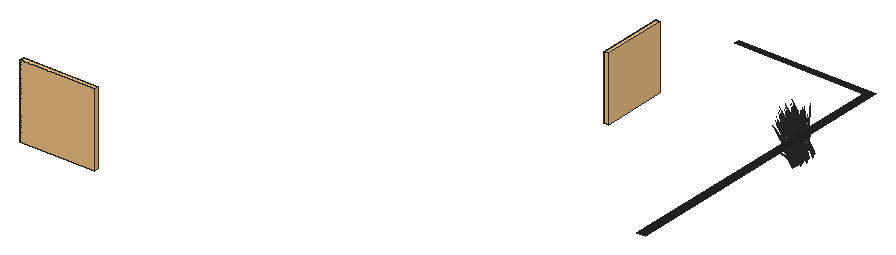
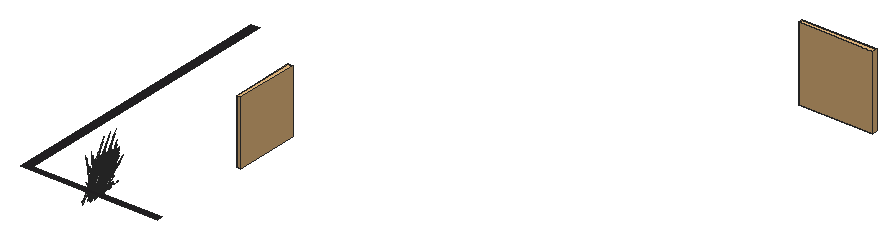
# SketchUp Ruby script. Lengths in inches.
U = 1.inch
M = Sketchup.active_model
def pt(a) = Geom::Point3d.new(a.map { |v| v * U })
def face(e, loops, mat)
  f = e.add_face(loops[0].map { |a| pt(a) })
  loops[1..].each { |l| e.add_face(l.map { |a| pt(a) }).erase! }
  f.material = f.back_material = mat if mat
  f
end
# faces: each face lists its corners as indices into pts; further lists are holes
def faces(e, pts, list, mat = nil) = list.each { |f| face(e, (f[0].is_a?(Array) ? f : [f]).map { |l| l.map { |i| pts[i] } }, mat) }
# xy, xz, yz: faces in a plane at the given z, y or x. An outline is a flat list of corners, or four numbers for a rectangle; further outlines are holes
def ring(l) = l.size == 4 ? [[l[0], l[1]], [l[2], l[1]], [l[2], l[3]], [l[0], l[3]]] : l.each_slice(2).to_a
def flat(e, list, mat, &to3) = list.each { |f| face(e, (f[0].is_a?(Array) ? f : [f]).map { |l| ring(l).map { |u, v| to3.(u, v) } }, mat) }
def xy(e, z, list, mat = nil) = flat(e, list, mat) { |x, y| [x, y, z] }
def xz(e, y, list, mat = nil) = flat(e, list, mat) { |x, z| [x, y, z] }
def yz(e, x, list, mat = nil) = flat(e, list, mat) { |y, z| [x, y, z] }
def lines(e, pts, list) = list.each { |a, b| e.add_line(pt(pts[a]), pt(pts[b])) }
# prism: a flat outline (further loops are holes) pulled along v
def prism(e, loops, v, mat = nil)
  f = face(e, loops, mat); d = Geom::Vector3d.new(v.map { |x| x * U })
  f.pushpull(f.normal.samedirection?(d) ? d.length : -d.length)
end
def box(e, o, s, mat = nil) = prism(e, [[o, [o[0] + s[0], o[1], o[2]], [o[0] + s[0], o[1] + s[1], o[2]], [o[0], o[1] + s[1], o[2]]]], [0, 0, s[2]], mat)
def at(x, y, z, deg = 0) = Geom::Transformation.translation(pt([x, y, z])) * Geom::Transformation.rotation(ORIGIN, Z_AXIS, deg.degrees)
def axes(o, x, y, z) = Geom::Transformation.new([*x, 0, *y, 0, *z, 0, *pt(o).to_a, 1])
def part(name) = M.definitions.add(name)
# library, detail: a bought-in or finely detailed component or shape, given as its bounding box
def library(name, o, s) = part(name).tap { |d| box(d.entities, o, s) }
def detail(e, o, s) = box(e.add_group.entities, o, s)
def put(e, d, t, mat = nil) = e.add_instance(d, t).tap { |i| i.material = mat if mat }
def group(e, t, mat = nil) = e.add_group.tap { |g| g.transformation = t; g.material = mat if mat }.entities
root = M.entities
M.materials.add("LightPink_Translucent").color = [144, 107, 117]
M.materials["LightPink_Translucent"].alpha = 0.75
M.materials.add("Marble_07_1K").color = [36, 34, 36]
c1 = library("mesh-163",[-551.08,-704.17,-20.03],[1929.24,1401.85,86.96])
c2 = part("Group11")
put(c2.entities,c1,at(0,0,0))
c3 = part("blade")
p = [[2.15,0.21,22],[0,0.17,0],[0.09,0.45,0],[2.18,0.31,22],[2.29,0.31,22],[0.38,0.45,0],
  [2.48,0.24,33],[2.49,0.24,33],[2.48,0.22,33]]
faces(c3.entities,p,[[0,1,2,3],[4,5,2,3],[6,3,4,7],[8,0,3,6]])
c4 = part("seeds")
p = [[0.3,-0.1,1.38],[-0.01,-0.03,1.59],[-0.01,-0.03,0.03],[0.14,-0.07,-0.07],[0.29,-0.03,3],[0.15,0.01,3.11]]
faces(c4.entities,p,[[0,1,2,3],[1,0,4,5]],"LightPink_Translucent")
c5 = part("blade with seeds")
put(c5.entities,c3,at(0,0,0))
put(c5.entities,c4,axes([2.4,0.25,30.99],[1.5799,-0.05474,1.17369],[-0.12525,1.92788,0.29478],[-0.07173,-0.02425,1.56792]))
xy(root,300,[[699.71,144,706,144,706,360,603,360,603,356,699.71,356]],"Marble_07_1K")
put(root,c2,axes([385.5,9.94,323.29],[-0.02883,0,0],[0,0,0.03929],[0,0.03937,0]))
put(root,c2,axes([603.79,247.71,324.08],[0,0.02488,0],[0,0,0.0342],[0.03937,0,0]))
put(root,c5,axes([686.23,308.34,267.22],[0.14872,0.18332,1.42242],[-0.6872,0.15433,0.11501],[-0.15531,-0.28779,0.60807]))
put(root,c5,axes([686.68,306.86,267.91],[-0.01214,0.06844,1.47228],[-0.59861,0.24837,-0.13912],[-0.17615,-0.12696,0.26054]))
put(root,c5,axes([686.55,308.08,268.23],[0.72473,-0.14676,0.44623],[0.12578,0.57568,0.36794],[-0.17045,-0.16967,0.92337]))
put(root,c5,axes([685.84,307.56,266.3],[0.33937,0.19872,0.95334],[-0.49424,0.11946,0.70045],[-0.10575,-0.15273,0.20998]))
put(root,c5,axes([686.66,308.61,268.13],[-0.55475,-0.27598,-0.58968],[0.39425,-0.48361,0.07116],[-0.20099,-0.16478,0.83415]))
put(root,c5,axes([686.47,308.24,267.76],[-0.10048,-0.4599,-0.29394],[0.5744,-0.12144,0.37948],[-0.15428,-0.13179,0.72609]))
put(root,c5,axes([686.72,308.2,267.93],[0.29569,-0.36271,0.05337],[0.42107,0.21117,0.42015],[-0.13613,-0.11629,0.64067]))
put(root,c5,axes([685.23,308.91,267.22],[0.24166,0.09837,1.42242],[-0.50011,0.41269,0.11501],[-0.3117,-0.18617,0.60807]))
put(root,c5,axes([686.4,308.62,267.89],[-0.64198,0.13573,-0.42412],[-0.1123,-0.514,-0.32852],[-0.17243,-0.1473,0.81151]))
put(root,c5,axes([686.85,308.16,268.51],[-0.4342,0.54737,-0.11304],[-0.6288,-0.31535,-0.62743],[-0.21858,-0.15465,0.95337]))
put(root,c5,axes([685.1875,308.01,267.91],[-0.13998,-0.00403,1.45204],[-0.44565,0.40302,-0.22964],[-0.23779,-0.08235,0.11645]))
put(root,c5,axes([687.99,311.73,266.76],[0.56221,0.23024,1.25546],[-0.55078,0.49601,0.49647],[-0.2467,-0.29398,1.05249]))
put(root,c5,axes([686.81,308.62,268.19],[0.10048,0.4599,0.29394],[-0.5744,0.12144,-0.37948],[-0.15428,-0.13179,0.72609]))
put(root,c5,axes([685.09,308.92,268.23],[0.53728,-0.42137,0.44623],[0.46337,0.44748,0.36794],[-0.25207,-0.07773,0.92337]))
put(root,c5,axes([685.33,308.92,267.93],[0.03276,-0.43418,0.05337],[0.49468,0.0119,0.42015],[-0.18949,-0.04543,0.64067]))
put(root,c5,axes([685.14,309.05,267.76],[-0.37017,-0.35748,-0.29394],[0.42268,-0.3384,0.37948],[-0.21476,-0.05149,0.72609]))
put(root,c5,axes([685.53,309.29,268.13],[-0.65035,-0.01375,-0.58968],[0.04368,-0.5789,0.07116],[-0.27552,-0.06109,0.83415]))
put(root,c5,axes([686.65,313.28,267.22],[0.14872,0.18332,1.42242],[-0.6872,0.15433,0.11501],[-0.15531,-0.28779,0.60807]))
put(root,c5,axes([684.65,308.35,267.91],[0.04823,0.05698,1.47228],[-0.23252,0.51221,-0.13912],[-0.23548,0.00371,0.26054]))
put(root,c5,axes([685.32,309.41,267.89],[-0.47241,0.37822,-0.42412],[-0.41372,-0.39954,-0.32852],[-0.24002,-0.05755,0.81151]))
put(root,c5,axes([685.67,309.24,268.19],[0.37017,0.35748,0.29394],[-0.42268,0.3384,-0.37948],[-0.21476,-0.05149,0.72609]))
put(root,c5,axes([684.25,309.91,266.3],[0.41536,-0.04086,0.95334],[-0.26347,0.35999,0.70045],[-0.20525,-0.054,0.20998]))
put(root,c5,axes([685.56,309.01,268.18],[-0.03484,0.58066,-0.10093],[-0.65957,-0.01587,-0.56021],[-0.25402,-0.04034,0.85122]))
put(root,c5,axes([684.72,309.8125,267.22],[0.26985,-0.01293,1.42242],[-0.17902,0.56047,0.11501],[-0.38456,-0.03467,0.60807]))
put(root,c5,axes([687.11,311.81,267.91],[-0.01214,0.06844,1.47228],[-0.59861,0.24837,-0.13912],[-0.17615,-0.12696,0.26054]))
put(root,c5,axes([686.97,313.02,268.23],[0.72473,-0.14676,0.44623],[0.12578,0.57568,0.36794],[-0.17045,-0.16967,0.92337]))
put(root,c5,axes([686.27,312.5,266.3],[0.33937,0.19872,0.95334],[-0.49424,0.11946,0.70045],[-0.10575,-0.15273,0.20998]))
put(root,c5,axes([687.09,313.55,268.13],[-0.55475,-0.27598,-0.58968],[0.39425,-0.48361,0.07116],[-0.20099,-0.16478,0.83415]))
put(root,c5,axes([684.61,310.24,267.93],[0.18381,-0.5206,0.39842],[0.60429,0.17802,0.32852],[-0.23764,0.03129,0.82444]))
put(root,c5,axes([686.89,313.1875,267.76],[-0.10048,-0.4599,-0.29394],[0.5744,-0.12144,0.37948],[-0.15428,-0.13179,0.72609]))
put(root,c5,axes([684.57,310.1,267.93],[-0.23895,-0.38931,0.05337],[0.43573,-0.19055,0.42015],[-0.19208,0.0376,0.64067]))
put(root,c5,axes([685.66,313.85,267.22],[0.24166,0.09837,1.42242],[-0.50011,0.41269,0.11501],[-0.3117,-0.18617,0.60807]))
put(root,c5,axes([684.49,310.29,267.76],[-0.54068,-0.15928,-0.29394],[0.1577,-0.46469,0.37948],[-0.21769,0.04261,0.72609]))
put(root,c5,axes([686.83,313.57,267.89],[-0.64198,0.13573,-0.42412],[-0.1123,-0.514,-0.32852],[-0.17243,-0.1473,0.81151]))
put(root,c5,axes([687.27,313.11,268.51],[-0.4342,0.54737,-0.11304],[-0.6288,-0.31535,-0.62743],[-0.21858,-0.15465,0.95337]))
put(root,c5,axes([685.06,310.24,268.19],[0.54068,0.15928,0.29394],[-0.1577,0.46469,-0.37948],[-0.21769,0.04261,0.72609]))
put(root,c5,axes([685.61,312.95,267.91],[-0.13998,-0.00403,1.45204],[-0.44565,0.40302,-0.22964],[-0.23779,-0.08235,0.11645]))
put(root,c5,axes([686.13,310.22,266.77],[0.18493,-0.0826,1.46963],[0.06377,0.5767,0.11501],[-0.40056,0.07652,0.52526]))
put(root,c5,axes([688.41,316.67,266.76],[0.56221,0.23024,1.25546],[-0.55078,0.49601,0.49647],[-0.2467,-0.29398,1.05249]))
put(root,c5,axes([687.23,313.5625,268.19],[0.10048,0.4599,0.29394],[-0.5744,0.12144,-0.37948],[-0.15428,-0.13179,0.72609]))
put(root,c5,axes([685.51,313.86,268.23],[0.53728,-0.42137,0.44623],[0.46337,0.44748,0.36794],[-0.25207,-0.07773,0.92337]))
put(root,c5,axes([684.15,310.6,267.91],[-0.10624,0.07413,1.45204],[0.00904,0.54162,-0.22964],[-0.24352,0.07044,0.11645]))
put(root,c5,axes([684.86,310.53,267.89],[-0.17625,0.51936,-0.42412],[-0.60429,-0.17802,-0.32852],[-0.2433,0.04762,0.81151]))
put(root,c5,axes([684.83,310.09,268.18],[0.32734,0.51701,-0.10093],[-0.58097,0.25407,-0.56021],[-0.24483,0.06821,0.85122]))
put(root,c5,axes([685.75,313.86,267.93],[0.03276,-0.43418,0.05337],[0.49468,0.0119,0.42015],[-0.18949,-0.04543,0.64067]))
put(root,c5,axes([685.5625,314,267.76],[-0.37017,-0.35748,-0.29394],[0.42268,-0.3384,0.37948],[-0.21476,-0.05149,0.72609]))
put(root,c5,axes([685.95,314.23,268.13],[-0.65035,-0.01375,-0.58968],[0.04368,-0.5789,0.07116],[-0.27552,-0.06109,0.83415]))
put(root,c5,axes([684.76,311.53,267.93],[-0.16135,-0.52549,0.39842],[0.63294,-0.0912,0.32852],[-0.18654,0.12359,0.82444]))
put(root,c5,axes([684.63,311.43,267.93],[-0.44663,-0.24013,0.05337],[0.26003,-0.34195,0.42015],[-0.14319,0.11055,0.64067]))
put(root,c5,axes([684.84,310.8,267.22],[0.22574,-0.12077,1.42242],[0.19004,0.55807,0.11501],[-0.35439,0.12613,0.60807]))
put(root,c5,axes([685.07,313.29,267.91],[0.04823,0.05698,1.47228],[-0.23252,0.51221,-0.13912],[-0.23548,0.00371,0.26054]))
put(root,c5,axes([685.15,311.36,268.19],[0.56631,-0.0816,0.29394],[0.14954,0.46647,-0.37948],[-0.16229,0.12529,0.72609]))
put(root,c5,axes([682.97,311.15,267.91],[0.08303,0.01531,1.47228],[0.25685,0.50448,-0.13912],[-0.16996,0.13241,0.26054]))
put(root,c5,axes([685.74,314.35,267.89],[-0.47241,0.37822,-0.42412],[-0.41372,-0.39954,-0.32852],[-0.24002,-0.05755,0.81151]))
put(root,c5,axes([683.66,312.75,266.3],[0.27113,-0.25877,0.95334],[0.10699,0.40966,0.70045],[-0.19594,0.07335,0.20998]))
put(root,c5,axes([686.09,314.18,268.19],[0.37017,0.35748,0.29394],[-0.42268,0.3384,-0.37948],[-0.21476,-0.05149,0.72609]))
put(root,c5,axes([684.67,314.85,266.3],[0.41536,-0.04086,0.95334],[-0.26347,0.35999,0.70045],[-0.20525,-0.054,0.20998]))
put(root,c5,axes([684.69,311.63,267.76],[-0.56631,0.0816,-0.29394],[-0.14954,-0.46647,0.37948],[-0.16229,0.12529,0.72609]))
put(root,c5,axes([685.99,313.95,268.18],[-0.03484,0.58066,-0.10093],[-0.65957,-0.01587,-0.56021],[-0.25402,-0.04034,0.85122]))
put(root,c5,axes([685.15,314.75,267.22],[0.26985,-0.01293,1.42242],[-0.17902,0.56047,0.11501],[-0.38456,-0.03467,0.60807]))
put(root,c5,axes([683.86,312.68,268.6875],[0.5741,0.15241,-0.05385],[-0.1766,0.46909,-0.24415],[-0.0939,0.07122,0.8053]))
put(root,c5,axes([684.85,311.31,268.18],[0.60181,0.31483,-0.10093],[-0.34671,0.45593,-0.56021],[-0.17003,0.15849,0.85122]))
put(root,c5,axes([686.2,319.82,267.22],[0.14872,0.18332,1.42242],[-0.6872,0.15433,0.11501],[-0.15531,-0.28779,0.60807]))
put(root,c5,axes([685.66,311.17,267.22],[0.1625,-0.17544,1.42242],[0.41029,0.47354,0.11501],[-0.28141,0.21565,0.60807]))
put(root,c5,axes([685.15,311.6875,267.89],[0.16713,0.52135,-0.42412],[-0.63294,0.0912,-0.32852],[-0.18138,0.14003,0.81151]))
put(root,c5,axes([685.04,315.18,267.93],[0.18381,-0.5206,0.39842],[0.60429,0.17802,0.32852],[-0.23764,0.03129,0.82444]))
put(root,c5,axes([684.99,315.04,267.93],[-0.23895,-0.38931,0.05337],[0.43573,-0.19055,0.42015],[-0.19208,0.0376,0.64067]))
put(root,c5,axes([685.51,312.56,267.93],[-0.53464,-0.0266,0.05337],[0.01466,-0.40172,0.42015],[-0.05594,0.15388,0.64067]))
put(root,c5,axes([685.68,312.6,267.93],[-0.46327,-0.38957,0.39842],[0.49199,-0.33598,0.32852],[-0.08546,0.18277,0.82444]))
put(root,c5,axes([684.91,315.24,267.76],[-0.54068,-0.15928,-0.29394],[0.1577,-0.46469,0.37948],[-0.21769,0.04261,0.72609]))
put(root,c5,axes([685.54,311.61,267.22],[0.12114,-0.19625,1.42242],[0.50818,0.40613,0.11501],[-0.22925,0.25313,0.60807]))
put(root,c5,axes([686.65,318.35,267.91],[-0.01214,0.06844,1.47228],[-0.59861,0.24837,-0.13912],[-0.17615,-0.12696,0.26054]))
put(root,c5,axes([685.68,312.71,267.76],[-0.4402,0.30062,-0.29394],[-0.41671,-0.34326,0.37948],[-0.0634,0.1744,0.72609]))
put(root,c5,axes([684.16,312.625,267.91],[-0.01617,0.11299,1.45204],[0.45894,0.39307,-0.22964],[-0.12015,0.18588,0.11645]))
put(root,c5,axes([685.48,315.18,268.19],[0.54068,0.15928,0.29394],[-0.1577,0.46469,-0.37948],[-0.21769,0.04261,0.72609]))
put(root,c5,axes([685.96,313.88,266.3],[-0.01684,-0.3395,0.95334],[0.42072,0.24214,0.70045],[-0.08274,0.16182,0.20998]))
put(root,c5,axes([686.52,319.5625,268.23],[0.72473,-0.14676,0.44623],[0.12578,0.57568,0.36794],[-0.17045,-0.16967,0.92337]))
put(root,c5,axes([686.56,315.16,266.77],[0.18493,-0.0826,1.46963],[0.06377,0.5767,0.11501],[-0.40056,0.07652,0.52526]))
put(root,c5,axes([685.81,319.04,266.3],[0.33937,0.19872,0.95334],[-0.49424,0.11946,0.70045],[-0.10575,-0.15273,0.20998]))
put(root,c5,axes([686.63,320.09,268.13],[-0.55475,-0.27598,-0.58968],[0.39425,-0.48361,0.07116],[-0.20099,-0.16478,0.83415]))
put(root,c5,axes([686.4375,319.73,267.76],[-0.10048,-0.4599,-0.29394],[0.5744,-0.12144,0.37948],[-0.15428,-0.13179,0.72609]))
put(root,c5,axes([684.57,315.54,267.91],[-0.10624,0.07413,1.45204],[0.00904,0.54162,-0.22964],[-0.24352,0.07044,0.11645]))
put(root,c5,axes([685.28,315.47,267.89],[-0.17625,0.51936,-0.42412],[-0.60429,-0.17802,-0.32852],[-0.2433,0.04762,0.81151]))
put(root,c5,axes([685.25,315.03,268.18],[0.32734,0.51701,-0.10093],[-0.58097,0.25407,-0.56021],[-0.24483,0.06821,0.85122]))
put(root,c5,axes([686.69,319.69,267.93],[0.29569,-0.36271,0.05337],[0.42107,0.21117,0.42015],[-0.13613,-0.11629,0.64067]))
put(root,c5,axes([685.98,312.4,268.43],[-0.01693,0.52814,-0.65454],[-0.71285,-0.03547,0.07899],[-0.07523,0.22375,0.92591]))
put(root,c5,axes([684.11,313.78,267.91],[0.07381,-0.03447,1.47228],[0.61004,0.22929,-0.13912],[-0.01434,0.19091,0.26054]))
put(root,c5,axes([685.2,320.4,267.22],[0.24166,0.09837,1.42242],[-0.50011,0.41269,0.11501],[-0.3117,-0.18617,0.60807]))
put(root,c5,axes([686.37,320.11,267.89],[-0.64198,0.13573,-0.42412],[-0.1123,-0.514,-0.32852],[-0.17243,-0.1473,0.81151]))
put(root,c5,axes([686.82,319.65,268.51],[-0.4342,0.54737,-0.11304],[-0.6288,-0.31535,-0.62743],[-0.21858,-0.15465,0.95337]))
put(root,c5,axes([685.18,316.47,267.93],[-0.16135,-0.52549,0.39842],[0.63294,-0.0912,0.32852],[-0.18654,0.12359,0.82444]))
put(root,c5,axes([685.06,316.375,267.93],[-0.44663,-0.24013,0.05337],[0.26003,-0.34195,0.42015],[-0.14319,0.11055,0.64067]))
put(root,c5,axes([685.26,315.74,267.22],[0.22574,-0.12077,1.42242],[0.19004,0.55807,0.11501],[-0.35439,0.12613,0.60807]))
put(root,c5,axes([685.15,319.49,267.91],[-0.13998,-0.00403,1.45204],[-0.44565,0.40302,-0.22964],[-0.23779,-0.08235,0.11645]))
put(root,c5,axes([687.96,323.21,266.76],[0.56221,0.23024,1.25546],[-0.55078,0.49601,0.49647],[-0.2467,-0.29398,1.05249]))
put(root,c5,axes([686.78,320.1,268.19],[0.10048,0.4599,0.29394],[-0.5744,0.12144,-0.37948],[-0.15428,-0.13179,0.72609]))
put(root,c5,axes([685.74,313.14,266.79],[0.01429,-0.29475,1.28107],[0.64291,0.15569,0.17703],[-0.0557,0.31414,0.60492]))
put(root,c5,axes([685.05,320.4,268.23],[0.53728,-0.42137,0.44623],[0.46337,0.44748,0.36794],[-0.25207,-0.07773,0.92337]))
put(root,c5,axes([685.57,316.3,268.19],[0.56631,-0.0816,0.29394],[0.14954,0.46647,-0.37948],[-0.16229,0.12529,0.72609]))
put(root,c5,axes([683.39,316.09,267.91],[0.08303,0.01531,1.47228],[0.25685,0.50448,-0.13912],[-0.16996,0.13241,0.26054]))
put(root,c5,axes([684.09,317.69,266.3],[0.27113,-0.25877,0.95334],[0.10699,0.40966,0.70045],[-0.19594,0.07335,0.20998]))
put(root,c5,axes([685.11,316.58,267.76],[-0.56631,0.0816,-0.29394],[-0.14954,-0.46647,0.37948],[-0.16229,0.12529,0.72609]))
put(root,c5,axes([685.3,320.4,267.93],[0.03276,-0.43418,0.05337],[0.49468,0.0119,0.42015],[-0.18949,-0.04543,0.64067]))
put(root,c5,axes([685.11,320.54,267.76],[-0.37017,-0.35748,-0.29394],[0.42268,-0.3384,0.37948],[-0.21476,-0.05149,0.72609]))
put(root,c5,axes([684.28,317.625,268.6875],[0.5741,0.15241,-0.05385],[-0.1766,0.46909,-0.24415],[-0.0939,0.07122,0.8053]))
put(root,c5,axes([685.5,320.77,268.13],[-0.65035,-0.01375,-0.58968],[0.04368,-0.5789,0.07116],[-0.27552,-0.06109,0.83415]))
put(root,c5,axes([685.28,316.26,268.18],[0.60181,0.31483,-0.10093],[-0.34671,0.45593,-0.56021],[-0.17003,0.15849,0.85122]))
put(root,c5,axes([686.09,316.12,267.22],[0.1625,-0.17544,1.42242],[0.41029,0.47354,0.11501],[-0.28141,0.21565,0.60807]))
put(root,c5,axes([685.57,316.63,267.89],[0.16713,0.52135,-0.42412],[-0.63294,0.0912,-0.32852],[-0.18138,0.14003,0.81151]))
put(root,c5,axes([684.62,319.83,267.91],[0.04823,0.05698,1.47228],[-0.23252,0.51221,-0.13912],[-0.23548,0.00371,0.26054]))
put(root,c5,axes([685.93,317.5,267.93],[-0.53464,-0.0266,0.05337],[0.01466,-0.40172,0.42015],[-0.05594,0.15388,0.64067]))
put(root,c5,axes([686.11,317.54,267.93],[-0.46327,-0.38957,0.39842],[0.49199,-0.33598,0.32852],[-0.08546,0.18277,0.82444]))
put(root,c5,axes([685.28,320.89,267.89],[-0.47241,0.37822,-0.42412],[-0.41372,-0.39954,-0.32852],[-0.24002,-0.05755,0.81151]))
put(root,c5,axes([685.63,320.72,268.19],[0.37017,0.35748,0.29394],[-0.42268,0.3384,-0.37948],[-0.21476,-0.05149,0.72609]))
put(root,c5,axes([684.22,321.39,266.3],[0.41536,-0.04086,0.95334],[-0.26347,0.35999,0.70045],[-0.20525,-0.054,0.20998]))
put(root,c5,axes([685.53,320.5,268.18],[-0.03484,0.58066,-0.10093],[-0.65957,-0.01587,-0.56021],[-0.25402,-0.04034,0.85122]))
put(root,c5,axes([684.69,321.3,267.22],[0.26985,-0.01293,1.42242],[-0.17902,0.56047,0.11501],[-0.38456,-0.03467,0.60807]))
put(root,c5,axes([685.96,316.55,267.22],[0.12114,-0.19625,1.42242],[0.50818,0.40613,0.11501],[-0.22925,0.25313,0.60807]))
put(root,c5,axes([686.1,317.66,267.76],[-0.4402,0.30062,-0.29394],[-0.41671,-0.34326,0.37948],[-0.0634,0.1744,0.72609]))
put(root,c5,axes([684.59,317.57,267.91],[-0.01617,0.11299,1.45204],[0.45894,0.39307,-0.22964],[-0.12015,0.18588,0.11645]))
put(root,c5,axes([686.38,318.82,266.3],[-0.01684,-0.3395,0.95334],[0.42072,0.24214,0.70045],[-0.08274,0.16182,0.20998]))
put(root,c5,axes([684.58,321.72,267.93],[0.18381,-0.5206,0.39842],[0.60429,0.17802,0.32852],[-0.23764,0.03129,0.82444]))
put(root,c5,axes([684.53,321.58,267.93],[-0.23895,-0.38931,0.05337],[0.43573,-0.19055,0.42015],[-0.19208,0.0376,0.64067]))
put(root,c5,axes([686.4,317.34,268.43],[-0.01693,0.52814,-0.65454],[-0.71285,-0.03547,0.07899],[-0.07523,0.22375,0.92591]))
put(root,c5,axes([684.53,318.73,267.91],[0.07381,-0.03447,1.47228],[0.61004,0.22929,-0.13912],[-0.01434,0.19091,0.26054]))
put(root,c5,axes([684.45,321.78,267.76],[-0.54068,-0.15928,-0.29394],[0.1577,-0.46469,0.37948],[-0.21769,0.04261,0.72609]))
put(root,c5,axes([685.02,321.73,268.19],[0.54068,0.15928,0.29394],[-0.1577,0.46469,-0.37948],[-0.21769,0.04261,0.72609]))
put(root,c5,axes([686.1,321.7,266.77],[0.18493,-0.0826,1.46963],[0.06377,0.5767,0.11501],[-0.40056,0.07652,0.52526]))
put(root,c5,axes([685.14,328.02,267.22],[0.14872,0.18332,1.42242],[-0.6872,0.15433,0.11501],[-0.15531,-0.28779,0.60807]))
put(root,c5,axes([686.28,326.81,267.91],[-0.09951,-0.08005,1.45204],[-0.66407,0.05075,-0.22964],[-0.10598,-0.19148,0.11645]))
